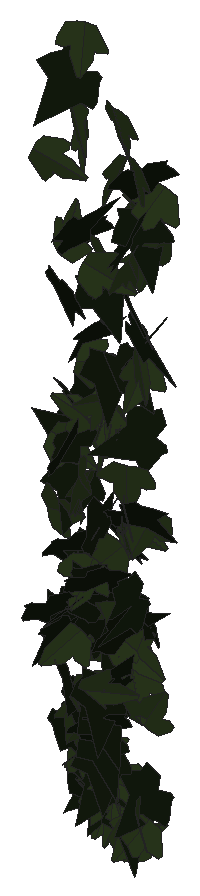
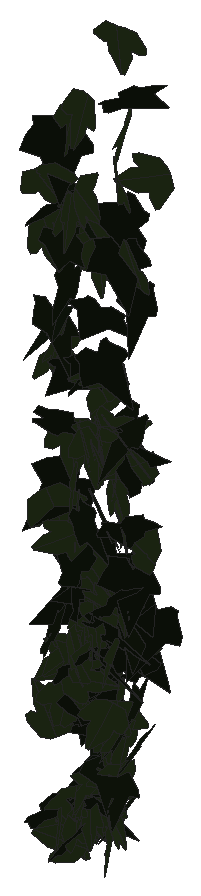
# SketchUp Ruby script. Lengths in inches.
U = 1.inch
M = Sketchup.active_model
def pt(a) = Geom::Point3d.new(a.map { |v| v * U })
def face(e, loops, mat)
  f = e.add_face(loops[0].map { |a| pt(a) })
  loops[1..].each { |l| e.add_face(l.map { |a| pt(a) }).erase! }
  f.material = f.back_material = mat if mat
  f
end
# faces: each face lists its corners as indices into pts; further lists are holes
def faces(e, pts, list, mat = nil) = list.each { |f| face(e, (f[0].is_a?(Array) ? f : [f]).map { |l| l.map { |i| pts[i] } }, mat) }
# xy, xz, yz: faces in a plane at the given z, y or x. An outline is a flat list of corners, or four numbers for a rectangle; further outlines are holes
def ring(l) = l.size == 4 ? [[l[0], l[1]], [l[2], l[1]], [l[2], l[3]], [l[0], l[3]]] : l.each_slice(2).to_a
def flat(e, list, mat, &to3) = list.each { |f| face(e, (f[0].is_a?(Array) ? f : [f]).map { |l| ring(l).map { |u, v| to3.(u, v) } }, mat) }
def xy(e, z, list, mat = nil) = flat(e, list, mat) { |x, y| [x, y, z] }
def xz(e, y, list, mat = nil) = flat(e, list, mat) { |x, z| [x, y, z] }
def yz(e, x, list, mat = nil) = flat(e, list, mat) { |y, z| [x, y, z] }
def lines(e, pts, list) = list.each { |a, b| e.add_line(pt(pts[a]), pt(pts[b])) }
# prism: a flat outline (further loops are holes) pulled along v
def prism(e, loops, v, mat = nil)
  f = face(e, loops, mat); d = Geom::Vector3d.new(v.map { |x| x * U })
  f.pushpull(f.normal.samedirection?(d) ? d.length : -d.length)
end
def box(e, o, s, mat = nil) = prism(e, [[o, [o[0] + s[0], o[1], o[2]], [o[0] + s[0], o[1] + s[1], o[2]], [o[0], o[1] + s[1], o[2]]]], [0, 0, s[2]], mat)
def at(x, y, z, deg = 0) = Geom::Transformation.translation(pt([x, y, z])) * Geom::Transformation.rotation(ORIGIN, Z_AXIS, deg.degrees)
def axes(o, x, y, z) = Geom::Transformation.new([*x, 0, *y, 0, *z, 0, *pt(o).to_a, 1])
def part(name) = M.definitions.add(name)
# library, detail: a bought-in or finely detailed component or shape, given as its bounding box
def library(name, o, s) = part(name).tap { |d| box(d.entities, o, s) }
def detail(e, o, s) = box(e.add_group.entities, o, s)
def put(e, d, t, mat = nil) = e.add_instance(d, t).tap { |i| i.material = mat if mat }
def group(e, t, mat = nil) = e.add_group.tap { |g| g.transformation = t; g.material = mat if mat }.entities
root = M.entities
M.materials.add("efeu1").color = [18, 25, 13]
M.materials.add("efeu2").color = [43, 57, 29]
c1 = part("ivyleaf_10")
p = [[0,0.5,-0.03],[-0.0625,2.02,-0.43],[-0.19,2.01,-0.46],[-0.54,1.05,-0.29],[-0.52,0.625,-0.18],[-0.83,0.76,-0.28],
  [-1.16,0.64,-0.33],[-1.15,0.33,-0.24],[-0.77,-0.39,0.02],[-0.3,-0.51,0.16],[0.04,-0.48,0.23],[-0.02,2.01,-0.4375],
  [-0.06,2.01,-0.43],[0.04,-0.49,0.23],[0.67,-0.49,0.14],[1.38,0.36,-0.2],[1.375,0.51,-0.24],[0.81,0.65,-0.19],
  [0.62,0.59,-0.15],[0.6,1.09,-0.28],[0.5,1.23,-0.31]]
faces(c1.entities,p,[[0,1,2,3,4,5,6,7,8,9,10],[11,12,0,13,14,15,16,17,18,19,20]],"efeu2")
c2 = part("ivyleaf_9")
p = [[1.54,2.16,1.25],[1.36,2.04,1.19],[-0.21,0.99,0.68],[-0.71,1.11,0.82],[-0.85,0.86,0.67],[-0.8,0.17,0.21],
  [-0.9,-0.01,0.1],[-0.67,-0.16,-0.02],[-0.08,-0.08,-0.05],[-0.03,-0.6,-0.4],[0.65,-0.88,-0.66],[0.83,-0.6,-0.49],
  [1.29,-0.42,-0.43],[1.8125,-0.07,-0.26],[1.21,0.44,0.15]]
faces(c2.entities,p,[[0,1,2,3,4,5,6,7,8,9,10,11,12,13,14]],"efeu1")
put(root,c1,axes([507.51,130.12,222.42],[0.22369,-0.65508,-0.6532],[-0.01958,0.66852,-0.67715],[0.92489,0.17259,0.14364]))
put(root,c2,axes([506.02,130.04,216.32],[0.60327,0.76951,-0.01236],[-0.00715,-0.00987,-0.98891],[-0.83114,0.55863,-0.00046]))
put(root,c1,axes([509.64,130.55,223.23],[-0.82502,-0.39058,0.08448],[-0.06465,-0.06079,-0.9124],[0.39435,-0.8271,0.02716]))
put(root,c1,axes([506.67,130.72,214.79],[0.69739,0.18415,-0.55324],[-0.5675,-0.09322,-0.69692],[-0.21809,0.83142,0.04439]))
put(root,c1,axes([508.18,130.22,231.99],[0.39072,0.16801,0.81133],[0.60185,0.55992,-0.39418],[-0.6169,0.65267,0.1293]))
put(root,c2,axes([506.55,130.75,215.38],[-0.1982,0.59517,-0.61915],[0.01996,-0.60633,-0.63633],[-0.90895,-0.14309,0.12104]))
put(root,c2,axes([509.86,130.81,217.56],[-0.94925,0.15868,-0.16544],[0.16908,-0.02821,-0.92887],[-0.17406,-0.89277,-0.00005]))
put(root,c2,axes([507.9375,130.11,218.125],[0.67293,0.70087,0.08749],[0.00907,0.10485,-0.97308],[-0.76232,0.61993,0.06566]))
put(root,c1,axes([507.39,130.79,218.08],[0.91343,0.05819,-0.21679],[-0.21748,0.00472,-0.9151],[-0.05552,0.93879,0.01803]))
put(root,c2,axes([506.13,130.75,222.5],[0.21897,0.66725,0.47312],[-0.17995,-0.42439,0.72459],[0.85342,-0.26069,0.03139]))
put(root,c2,axes([506.1,131.37,212.26],[0.11327,-0.51373,0.7615],[0.14559,-0.74753,-0.52596],[0.90697,0.18415,-0.01068]))
put(root,c2,axes([509.71,130.59,233.71],[-0.65043,0.71816,-0.07996],[0.06542,-0.04953,-0.97463],[-0.77729,-0.60512,-0.01512]))
put(root,c2,axes([507.82,131.23,212.61],[-0.01869,-0.91445,0.14545],[-0.03055,-0.13929,-0.95084],[0.99863,-0.02138,-0.02636]))
put(root,c2,axes([506.8,130.22,232.93],[0.13148,0.80663,-0.34036],[-0.07517,0.33842,0.84054],[0.93712,-0.08602,0.11518]))
put(root,c2,axes([508.11,130.6,211.57],[0.21677,0.75126,-0.35187],[-0.18918,-0.30137,-0.804],[-0.86951,0.25286,0.08721]))
put(root,c1,axes([505.3125,130.74,235.96],[-0.39317,0.00444,-0.83669],[0.86879,-0.01039,-0.37864],[-0.0122,-0.88298,0.00025]))
put(root,c2,axes([506.23,130.58,230.54],[0.73231,0.01794,-0.58013],[-0.60177,-0.02828,-0.70535],[-0.03436,0.87757,-0.01087]))
put(root,c2,axes([507.98,130.97,212.01],[0.1134,-0.78751,-0.35504],[-0.06745,0.34892,-0.79549],[0.86121,0.13102,-0.01555]))
put(root,c1,axes([507.64,131.52,225.35],[-0.10453,-0.15557,-0.82876],[-0.30374,-0.74642,0.18707],[-0.8226,0.29538,0.03624]))
put(root,c2,axes([506.73,130.43,216.23],[0.04802,0.84119,0.20336],[-0.12416,0.19982,-0.8668],[-0.9244,0.01686,0.12698]))
put(root,c1,axes([507.04,131.14,221.83],[0.11652,-0.80477,0.07546],[0.00151,-0.07302,-0.84441],[0.87268,0.10758,-0.00861]))
put(root,c2,axes([506.61,131.2,214.37],[0.57647,0.01295,0.73475],[-0.73249,0.08515,0.5732],[-0.05904,-0.93002,0.06271]))
put(root,c1,axes([507.84,130.46,212.82],[0.2376,-0.0265,0.91181],[0.44317,0.802,-0.08187],[-0.83726,0.41698,0.21541]))
put(root,c2,axes([506.0625,130.98,210.82],[0.6123,-0.62848,-0.31639],[-0.15418,0.27927,-0.87669],[0.73817,0.57965,0.07933]))
put(root,c1,axes([509.5625,130.74,232.48],[-0.12268,-0.76915,-0.51986],[0.04515,0.49882,-0.80812],[0.98966,-0.1181,-0.02757]))
put(root,c2,axes([506.8,130.93,223.39],[-0.23719,0.24096,0.7891],[-0.72343,0.36942,-0.32365],[-0.46463,-0.69819,0.10109]))
put(root,c1,axes([506.87,131.11,241.73],[0.92982,0.07915,0.05534],[0.05069,0.06904,-0.89666],[-0.08966,0.85982,0.0669]))
put(root,c2,axes([509.03,130.27,216.1],[-0.12891,0.48678,-0.84003],[-0.15685,0.82583,0.50262],[0.95812,0.20069,-0.03074]))
put(root,c2,axes([506.24,131.78,239.47],[-0.64566,-0.6745,0.29511],[-0.10722,-0.30219,-0.92526],[0.72838,-0.64238,0.12539]))
put(root,c2,axes([508.16,130.51,219.97],[-0.10919,0.43978,0.84541],[-0.32641,0.7822,-0.44906],[-0.89531,-0.33881,0.06061]))
put(root,c1,axes([509.59,130.92,236.89],[-0.83081,0.51933,0.10522],[-0.09006,0.05729,-0.96528],[-0.56428,-0.77378,-0.00085]))
put(root,c2,axes([507.66,131.34,216.11],[0.49286,0.18158,0.73537],[-0.76588,-0.08775,0.49942],[0.18722,-0.83697,0.10718]))
put(root,c1,axes([509.41,130.75,221.4375],[-0.47529,0.59938,0.49368],[-0.39644,0.31041,-0.75853],[-0.6677,-0.61096,0.09895]))
put(root,c2,axes([507.15,130.6,217.41],[0.1547,0.25309,-0.90446],[0.32905,0.81571,0.29907],[0.92121,-0.33387,0.04506]))
put(root,c1,axes([507.09,131.08,211.97],[-0.4972,-0.78401,-0.15345],[0.08533,0.12759,-0.92837],[0.79432,-0.50445,0.00368]))
put(root,c1,axes([507.4,131.13,211.16],[-0.1041,-0.85,-0.1351],[0.0156,0.1342,-0.85635],[0.86053,-0.10526,-0.00082]))
put(root,c1,axes([505.92,130.94,223.29],[0.40684,0.21771,0.73353],[0.64621,0.37366,-0.4523],[-0.46685,0.70694,0.01317]))
put(root,c1,axes([507.17,131.3125,224.41],[0.35403,0.29869,0.74554],[-0.68712,-0.34292,0.45117],[0.48097,-0.70976,0.09576]))
put(root,c2,axes([507.78,131.78,208.44],[-0.56748,-0.59347,0.19389],[-0.05747,-0.20027,-0.81898],[0.66937,-0.52033,0.09407]))
put(root,c2,axes([509.32,130.75,221.28],[0.89176,0.40166,0.14597],[0.12141,0.08958,-0.9544],[-0.44319,0.83274,0.03226]))
put(root,c1,axes([506.56,131.13,237.94],[-0.36719,0.77603,-0.0306],[0.01766,-0.02496,-0.88112],[-0.83853,-0.34035,-0.00515]))
put(root,c2,axes([507.64,131.59,209.55],[-0.18421,-0.79563,-0.1231],[0.02792,0.11552,-0.84626],[0.86829,-0.17251,0.00109]))
put(root,c2,axes([507.78,131.68,226.88],[-0.01706,-0.83263,0.08311],[-0.00568,-0.07983,-0.86608],[0.90335,-0.01623,-0.00387]))
put(root,c1,axes([506.66,131.01,211.23],[-0.03055,0.89092,0.19113],[-0.12499,0.17885,-0.92023],[-0.97447,-0.05087,0.11204]))
put(root,c1,axes([505.24,131.38,219.68],[-0.34688,-0.0553,0.84168],[0.87555,0.00865,0.33522],[-0.03073,0.87067,0.05013]))
put(root,c1,axes([508.08,131.42,207.92],[0.80603,0.44235,-0.25922],[-0.2438,-0.10784,-0.90199],[-0.49118,0.77942,0.02232]))
put(root,c1,axes([509.14,130.94,220.37],[-0.52533,0.48217,0.55768],[-0.46845,0.31044,-0.70968],[-0.56925,-0.70044,0.06936]))
put(root,c2,axes([509.2,131.07,230.5625],[0.76083,-0.21108,-0.52246],[-0.51695,0.15267,-0.7648],[0.28123,0.85167,0.00761]))
put(root,c2,axes([507.49,131.57,210.23],[0.10488,-0.8054,-0.15631],[0.04078,0.15559,-0.84173],[0.88391,0.08839,0.05738]))
put(root,c2,axes([509.5,131.65,232.43],[-0.66022,0.52595,-0.43888],[0.10216,-0.52712,-0.78539],[-0.67735,-0.59216,0.30932]))
put(root,c2,axes([506.31,131.33,211.94],[0.67383,-0.57215,-0.32167],[-0.2202,0.23493,-0.87973],[0.66702,0.65555,0.03453]))
put(root,c2,axes([509.76,131.1,236.48],[0.30402,0.84312,-0.2646],[-0.08144,-0.24305,-0.92441],[-0.94763,0.29138,-0.00545]))
put(root,c1,axes([506.8,131.33,209.67],[0.24005,0.86441,0.10363],[0.0417,0.09294,-0.92812],[-0.93882,0.22515,-0.01473]))
put(root,c1,axes([509.4375,131.78,227.32],[0.31976,0.69185,-0.51929],[-0.22438,-0.45416,-0.78257],[-0.89374,0.36155,0.01067]))
put(root,c2,axes([509.375,131.84,233.8],[0.02467,-0.95225,-0.1035],[0.0857,0.10532,-0.94851],[0.95402,0.01517,0.08788]))
put(root,c1,axes([507.86,131.29,232.05],[-0.75962,0.19101,0.44917],[-0.44956,0.11517,-0.75797],[-0.24089,-0.81729,-0.00184]))
put(root,c1,axes([508.27,132.05,207.27],[-0.17892,-0.59799,0.64497],[0.15661,-0.64187,-0.6034],[0.91716,-0.00705,0.22886]))
put(root,c2,axes([507.67,131.47,212.4375],[0.63074,0.60527,0.15407],[-0.11719,-0.10116,0.8747],[0.6627,-0.59397,0.00803]))
put(root,c1,axes([507.28,131.67,208.72],[-0.62618,-0.56189,0.31978],[-0.21808,-0.23325,-0.83928],[0.65648,-0.61344,0.02621]))
put(root,c1,axes([509.77,131.74,220.66],[-0.6643,-0.56084,0.4009],[-0.23681,-0.33723,-0.86416],[0.64745,-0.69878,0.09527]))
put(root,c1,axes([507.96,131.44,217.64],[-0.87988,-0.07199,0.1179],[-0.11504,-0.03898,-0.88233],[0.07648,-0.88689,0.02921]))
put(root,c1,axes([507.6875,131.42,216.09],[-0.78788,-0.37149,-0.14448],[0.11884,0.08656,-0.87064],[0.38046,-0.79632,-0.02724]))
put(root,c1,axes([509.38,131.68,206.74],[0.78886,0.19333,-0.47778],[-0.49532,-0.05843,-0.78394],[-0.21077,0.86091,0.05409]))
put(root,c2,axes([506.33,131.76,208.04],[0.42163,-0.72424,-0.02675],[-0.00568,0.02639,-0.85563],[0.78265,0.39035,0.0082]))
put(root,c1,axes([506.57,131.52,217.37],[-0.76795,0.48721,0.15616],[-0.27701,-0.11916,-0.86109],[-0.47585,-0.71691,0.24926]))
put(root,c2,axes([509.78,131.9375,224.29],[-0.79418,-0.02153,0.46464],[-0.45882,-0.11469,-0.78956],[0.07637,-0.91294,0.08823]))
put(root,c1,axes([509.42,131.57,227.93],[-0.24669,0.86822,-0.1102],[0.00757,-0.1077,-0.93343],[-0.9446,-0.22761,0.0213]))
put(root,c2,axes([507.86,131.99,208.23],[-0.67659,-0.50348,-0.08342],[0.05916,0.05988,-0.83577],[0.54743,-0.62874,-0.01279]))
put(root,c2,axes([509.23,131.47,229.12],[0.80751,-0.47226,-0.30843],[-0.22573,0.22304,-0.93249],[0.51692,0.83514,0.07462]))
put(root,c1,axes([506.78,131.23,220.67],[-0.06121,0.23699,0.80567],[-0.7257,0.42004,-0.18476],[-0.48874,-0.65338,0.17345]))
put(root,c1,axes([509.86,131.85,232.65],[-0.31535,-0.82469,0.21343],[-0.0766,-0.1926,-0.90985],[0.91463,-0.30047,-0.00261]))
put(root,c2,axes([506.0625,131.33,218.63],[0.26967,0.76182,-0.1507],[-0.07172,-0.13066,-0.83345],[-0.83444,0.25743,0.02294]))
put(root,c1,axes([507.43,131.9,223.72],[0.61735,-0.52979,0.21101],[0.17285,-0.12574,-0.81038],[0.58781,0.59338,0.01668]))
put(root,c1,axes([508.32,131.55,238.33],[-0.86159,0.34972,0.01279],[-0.01186,0.00558,-0.9059],[-0.37774,-0.79784,-0.00073]))
put(root,c1,axes([508,131.68,218.68],[0.72526,-0.08054,-0.56334],[-0.56826,0.14274,-0.70047],[0.16398,0.85089,0.06419]))
put(root,c2,axes([506.02,131.27,225.22],[0.83651,0.00069,-0.4552],[-0.44144,0.23361,-0.81088],[0.11107,0.92325,0.20552]))
put(root,c1,axes([506.98,131.34,227.01],[-0.09575,-0.14743,-0.82124],[0.74954,0.38599,-0.15599],[0.43687,-0.69457,0.08763]))
put(root,c1,axes([505.6875,131.61,231.65],[0.93504,-0.24196,-0.07768],[0.08801,0.01431,0.93417],[-0.25893,-0.86887,0.03702]))
put(root,c1,axes([507.29,131.8,224.46],[0.81408,0.1794,0.20816],[0.20806,0.05499,-0.80578],[-0.20244,0.77796,0.00896]))
put(root,c2,axes([505.92,132.18,221.14],[-0.50736,-0.64947,-0.11852],[0.07707,0.08903,-0.83361],[0.70796,-0.47513,0.00581]))
put(root,c1,axes([507.42,131.75,224.69],[0.41217,-0.6592,-0.26695],[-0.11342,0.23563,-0.79172],[0.75554,0.39499,0.02678]))
put(root,c1,axes([506.74,131.99,216.98],[-0.00689,0.01853,-0.85876],[0.80273,-0.35997,-0.01437],[-0.38899,-0.74317,-0.01445]))
put(root,c2,axes([506.45,131.625,232.69],[0.14977,0.76368,-0.28576],[-0.09428,-0.2631,-0.80632],[-0.87145,0.15971,0.03812]))
put(root,c1,axes([509.46,131.48,207.25],[-0.49468,0.55899,0.53516],[-0.41586,0.34719,-0.74869],[-0.70737,-0.59502,0.0659]))
put(root,c2,axes([509.77,131.5,228.76],[-0.28349,0.85304,0.12785],[-0.06409,0.11032,-0.92787],[-0.92859,-0.26804,0.025]))
put(root,c2,axes([507.45,132.24,208.25],[-0.82597,-0.21596,0.15132],[-0.1563,-0.02278,-0.82629],[0.2338,-0.77817,-0.01781]))
put(root,c1,axes([507.35,131.89,224.24],[-0.83064,-0.4581,0.08244],[-0.07166,-0.04078,-0.94859],[0.45991,-0.83372,0.0011]))
put(root,c2,axes([507.22,131.98,214.77],[-0.77037,0.28188,0.14255],[-0.14258,0.03882,-0.79756],[-0.30702,-0.72532,0.01271]))
put(root,c1,axes([508.71,131.5,205.88],[-0.21565,-0.34276,0.78006],[0.35153,0.67632,0.41154],[-0.81833,0.38085,-0.02878]))
put(root,c1,axes([509.79,132.13,234.98],[0.81649,0.23327,-0.45699],[-0.4323,-0.14982,-0.84887],[-0.27634,0.92361,-0.02228]))
put(root,c2,axes([506.97,131.41,209.72],[0.04772,0.87142,0.22213],[-0.14053,0.2178,-0.8962],[-0.95875,0.01145,0.14241]))
put(root,c1,axes([507.94,131.83,208.43],[-0.38758,0.72921,0.00526],[-0.00624,0.00279,-0.84524],[-0.78754,-0.3589,0.00411]))
put(root,c2,axes([508.12,132.34,206.83],[0.15478,-0.86725,0.04547],[0.00869,-0.04299,-0.91418],[0.93778,0.14354,0.00096]))
put(root,c2,axes([508.02,131.93,227.17],[-0.08588,-0.46378,-0.70131],[0.42262,0.57351,-0.4582],[0.77632,-0.36352,0.17186]))
put(root,c1,axes([507.12,132.05,208.42],[0.82994,0.26145,-0.01909],[-0.01727,-0.00998,-0.84418],[-0.28254,0.76862,-0.00447]))
put(root,c2,axes([506.28,132.56,217.67],[-0.32853,-0.6843,0.26687],[-0.10754,-0.23655,-0.77881],[0.78194,-0.32004,0.00502]))
put(root,c1,axes([508.3,132.03,208.53],[0.3795,0.7887,-0.098],[-0.01442,-0.09716,-0.89753],[-0.85773,0.35059,-0.02827]))
put(root,c1,axes([506.86,131.87,212.45],[-0.71093,-0.30243,-0.30647],[0.28609,0.12926,-0.75337],[0.35515,-0.70954,-0.00661]))
put(root,c1,axes([507.95,132.03,224.24],[0.49933,-0.65146,-0.1673],[-0.07675,0.14672,-0.83034],[0.72063,0.46702,0.02749]))
put(root,c1,axes([508.16,131.62,215.68],[0.30307,-0.11484,-0.8045],[-0.44457,0.67709,-0.25984],[0.71812,0.46764,0.17867]))
put(root,c2,axes([506.98,132.18,230.17],[-0.34876,-0.40962,-0.64154],[0.52212,0.39313,-0.5347],[0.60577,-0.57468,0.09151]))
put(root,c1,axes([507.66,132.62,214.55],[-0.07919,0.11697,0.77184],[-0.12781,-0.73817,0.10884],[0.8013,-0.10618,0.09364]))
put(root,c2,axes([507.85,132.26,220.94],[-0.50719,0.48929,-0.40968],[0.28239,-0.29494,-0.70518],[-0.61685,-0.53733,0.01402]))
put(root,c2,axes([509.1875,132.85,207.82],[-0.39028,-0.69503,0.44921],[-0.20966,-0.39742,-0.79705],[0.80057,-0.44291,0.01026]))
put(root,c2,axes([507,132.22,228.18],[-0.21268,0.61985,-0.48244],[-0.03153,-0.48426,-0.66007],[-0.83555,-0.1395,0.1477]))
put(root,c2,axes([507.12,132.35,216.4],[-0.84092,0.11108,0.2626],[-0.2622,0.02004,-0.84811],[-0.11203,-0.88074,0.01382]))
put(root,c1,axes([507.89,132.58,213.88],[-0.13306,-0.06021,0.80532],[-0.49663,-0.62619,-0.12673],[0.676,-0.47189,0.06541]))
put(root,c2,axes([507.68,132.72,214.69],[-0.30214,-0.8678,0.1042],[-0.04704,-0.09394,-0.9188],[0.87277,-0.30548,-0.01345]))
put(root,c1,axes([506.02,132.55,208.44],[0.38395,-0.66756,0.38321],[0.1979,-0.31984,-0.7865],[0.79937,0.39982,0.01065]))
put(root,c1,axes([507.15,131.86,209.36],[0.33327,0.55847,0.51466],[0.24002,0.44242,-0.66338],[-0.76929,0.37998,0.01598]))
put(root,c1,axes([508.52,132.35,212.86],[-0.87511,-0.30233,-0.16111],[0.26308,-0.23783,-0.84237],[0.25572,-0.78993,0.31528]))
put(root,c2,axes([506.35,132.35,225.36],[-0.83628,0.29743,-0.1116],[0.10511,-0.04589,-0.86263],[-0.32492,-0.78039,0.00819]))
put(root,c1,axes([509.21,132.27,211.3],[-0.77166,-0.25719,0.42322],[0.40251,0.13078,0.81339],[-0.28852,0.87033,0.00284]))
put(root,c1,axes([508.5,132.03,234.1],[0.08404,-0.74463,-0.41053],[0.03978,0.39905,-0.77531],[0.90934,0.05136,0.07186]))
put(root,c2,axes([507.66,132.58,218.73],[0.20211,-0.37502,0.66584],[0.48424,-0.46893,-0.42197],[0.63848,0.47436,0.10926]))
put(root,c1,axes([508.26,131.88,214.71],[0.4026,0.35749,0.65954],[0.40162,0.51901,-0.53161],[-0.67592,0.52132,0.07698]))
put(root,c1,axes([507.36,132.23,216.73],[-0.78854,0.35253,0.19646],[-0.26966,-0.13942,-0.83218],[-0.30026,-0.8006,0.23143]))
put(root,c1,axes([508.08,132.4,215.34],[0.28554,-0.84895,0.02645],[0.01203,-0.02386,-0.89567],[0.84927,0.28577,0.0038]))
put(root,c1,axes([505.68,132.61,236.35],[0.59879,-0.39514,0.54166],[0.49021,-0.25882,-0.70674],[0.50815,0.71532,0.0435]))
put(root,c1,axes([507.42,132.74,235.22],[0.23265,-0.67836,0.50179],[0.1718,-0.45565,-0.74012],[0.88248,0.26754,0.0118]))
put(root,c1,axes([508.34,132.0625,214.31],[0.44743,0.31633,0.74532],[0.6402,0.40341,-0.54157],[-0.55309,0.72284,-0.02392]))
put(root,c2,axes([508.77,132.91,215.47],[0.02404,-0.37705,0.71049],[0.12571,-0.67419,-0.39093],[0.8333,0.11259,0.03848]))
put(root,c1,axes([507.47,132.29,208.26],[-0.80143,0.27357,0.17482],[-0.2167,-0.06462,-0.81182],[-0.27073,-0.75812,0.13229]))
put(root,c1,axes([506.32,132.08,215.62],[-0.34443,0.67504,0.28251],[-0.12241,0.24688,-0.77644],[-0.77626,-0.33844,-0.00291]))
put(root,c1,axes([508.36,132.3125,219.84],[-0.45146,-0.16581,-0.68793],[0.72905,0.00941,-0.44611],[0.10444,-0.78243,0.14042]))
put(root,c1,axes([506.63,131.98,207.27],[-0.32679,0.43601,0.57989],[-0.41608,0.40726,-0.54863],[-0.6413,-0.48642,0.06045]))
